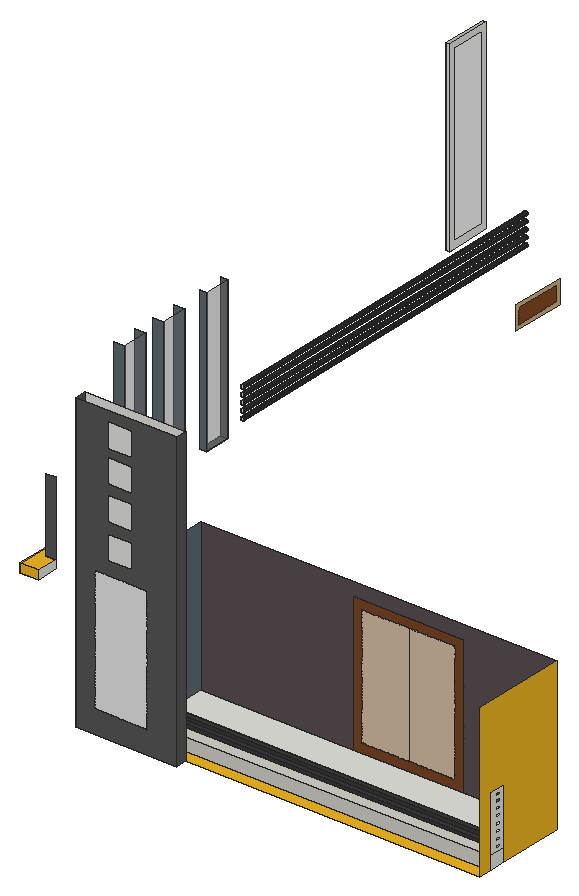
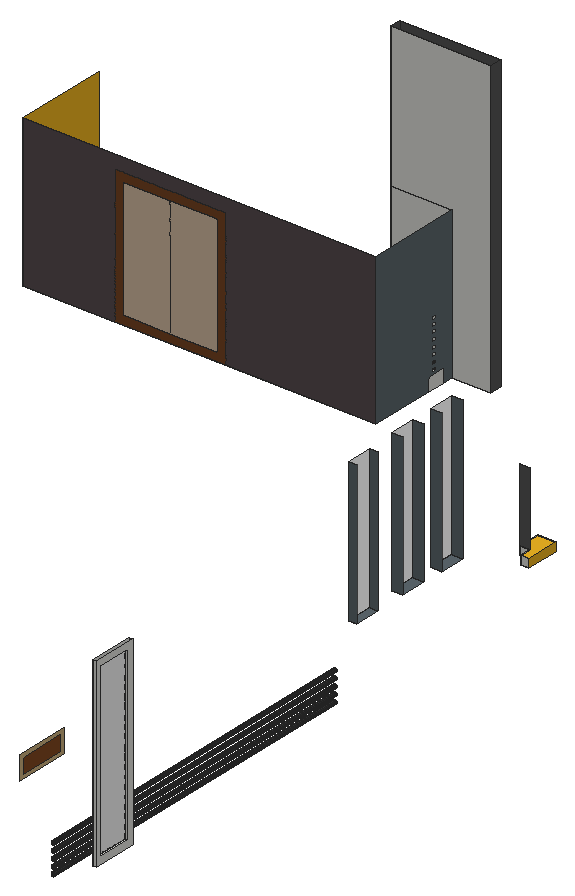
# SketchUp Ruby script. Lengths in inches.
U = 1.inch
M = Sketchup.active_model
def pt(a) = Geom::Point3d.new(a.map { |v| v * U })
def face(e, loops, mat)
  f = e.add_face(loops[0].map { |a| pt(a) })
  loops[1..].each { |l| e.add_face(l.map { |a| pt(a) }).erase! }
  f.material = f.back_material = mat if mat
  f
end
# faces: each face lists its corners as indices into pts; further lists are holes
def faces(e, pts, list, mat = nil) = list.each { |f| face(e, (f[0].is_a?(Array) ? f : [f]).map { |l| l.map { |i| pts[i] } }, mat) }
# xy, xz, yz: faces in a plane at the given z, y or x. An outline is a flat list of corners, or four numbers for a rectangle; further outlines are holes
def ring(l) = l.size == 4 ? [[l[0], l[1]], [l[2], l[1]], [l[2], l[3]], [l[0], l[3]]] : l.each_slice(2).to_a
def flat(e, list, mat, &to3) = list.each { |f| face(e, (f[0].is_a?(Array) ? f : [f]).map { |l| ring(l).map { |u, v| to3.(u, v) } }, mat) }
def xy(e, z, list, mat = nil) = flat(e, list, mat) { |x, y| [x, y, z] }
def xz(e, y, list, mat = nil) = flat(e, list, mat) { |x, z| [x, y, z] }
def yz(e, x, list, mat = nil) = flat(e, list, mat) { |y, z| [x, y, z] }
def lines(e, pts, list) = list.each { |a, b| e.add_line(pt(pts[a]), pt(pts[b])) }
# prism: a flat outline (further loops are holes) pulled along v
def prism(e, loops, v, mat = nil)
  f = face(e, loops, mat); d = Geom::Vector3d.new(v.map { |x| x * U })
  f.pushpull(f.normal.samedirection?(d) ? d.length : -d.length)
end
def box(e, o, s, mat = nil) = prism(e, [[o, [o[0] + s[0], o[1], o[2]], [o[0] + s[0], o[1] + s[1], o[2]], [o[0], o[1] + s[1], o[2]]]], [0, 0, s[2]], mat)
def at(x, y, z, deg = 0) = Geom::Transformation.translation(pt([x, y, z])) * Geom::Transformation.rotation(ORIGIN, Z_AXIS, deg.degrees)
def axes(o, x, y, z) = Geom::Transformation.new([*x, 0, *y, 0, *z, 0, *pt(o).to_a, 1])
def part(name) = M.definitions.add(name)
# library, detail: a bought-in or finely detailed component or shape, given as its bounding box
def library(name, o, s) = part(name).tap { |d| box(d.entities, o, s) }
def detail(e, o, s) = box(e.add_group.entities, o, s)
def put(e, d, t, mat = nil) = e.add_instance(d, t).tap { |i| i.material = mat if mat }
def group(e, t, mat = nil) = e.add_group.tap { |g| g.transformation = t; g.material = mat if mat }.entities
root = M.entities
M.materials.add("[0045_Goldenrod]").color = [239, 181, 35]
M.materials.add("[Asphalt New]").color = [89, 79, 82]
M.materials.add("[Color M06]").color = [86, 86, 86]
M.materials.add("[Color M07]").color = [58, 58, 58]
M.materials.add("[Formica Laminate Light]").color = [213, 189, 164]
M.materials.add("[Formica Speckled Grey]").color = [94, 105, 111]
M.materials.add("[Sketchy Siding Scale]").color = [229, 229, 229]
M.materials.add("[Sketchy Siding Scale]1").color = [244, 244, 244]
M.materials.add("[Tile Travertine 2 inch]").color = [211, 208, 201]
M.materials.add("[Translucent Glass Gray]1").color = [128, 128, 128]
M.materials["[Translucent Glass Gray]1"].alpha = 0.5
M.materials.add("[Wood Cherry Original]").color = [130, 73, 35]
M.materials.add("[Wood Floor Light]").color = [204, 176, 127]
M.materials.add("[Wood Veneer 01]1").color = [120, 70, 37]
xy(root,228.72,[[38.625,253.03,38.625,280.03,45.3125,280.03,45.3125,270.46,53.375,270.46,53.375,253.03]],"[0045_Goldenrod]")
xy(root,232.59,[[226.34,133.21,513.45,147.47],[226.34,147.47,513.45,200.74]])
xy(root,232.59,[[226.34,123.625,513.45,133.21]],"[0045_Goldenrod]")
xy(root,232.59,[[194.63,114.1875,276.16,123.625]],"[Color M06]")
xy(root,235.53,[[38.625,253.03,53.375,253.03,53.375,270.46,45.3125,270.46,45.3125,280.03,38.625,280.03]],"[0045_Goldenrod]")
xy(root,238.4,[[0,731.17,2.5625,767.73]])
xy(root,242.9,[[226.34,133.21,513.45,147.47]],"[Tile Travertine 2 inch]")
xy(root,244.23,[[0,735.45,2.5625,763.82]])
xy(root,245.27,[[226.34,139.81,513.45,143.95]])
xy(root,247.83,[[226.34,139.81,513.45,143.95]],"[Color M07]")
xy(root,250.64,[[226.34,139.81,513.45,143.95]])
xy(root,251.86,[[53.375,329.31,62.1875,350.56],[53.375,368.62,61.9375,389.87],[53.375,415.62,59.375,436.87]],"[Formica Speckled Grey]")
xy(root,253.2,[[226.34,139.81,513.45,143.95]],"[Color M07]")
xz(root,114.1875,[[[194.63,232.59,276.16,471],[209.79,250.99,251.85,351.68],[220.22,443.22,239.85,462.84],[220.22,362.15,239.85,381.78],[220.22,417.34,239.85,436.97],[220.22,390.15,239.85,409.78]]],"[Color M06]")
xz(root,114.1875,[[209.79,250.99,251.85,351.68]],"[Sketchy Siding Scale]")
xz(root,123.625,[[194.63,232.59,194.63,471,276.16,471,276.16,354.51,226.34,354.51,226.34,232.59],[226.34,232.59,276.16,354.51]])
xz(root,133.21,[[226.34,232.59,513.45,242.9]],"[Tile Travertine 2 inch]")
xz(root,139.81,[[226.34,245.27,513.45,247.83],[226.34,250.64,513.45,253.2]],"[Color M07]")
xz(root,143.95,[[226.34,245.27,513.45,247.83],[226.34,250.64,513.45,253.2]])
xz(root,147.47,[[226.34,232.59,513.45,242.9]])
xz(root,200.74,[[226.34,232.59,348.83,232.59,348.83,343.46,438.71,343.46,438.71,232.59,513.45,232.59,513.45,354.51,226.34,354.51]],"[Asphalt New]")
xz(root,200.74,[[355.93,239.69,393.77,336.36],[393.77,239.69,431.6,336.36]],"[Formica Laminate Light]")
xz(root,200.74,[[[348.83,232.59,438.71,343.46],[355.93,239.69,431.6,336.36]]],"[Wood Veneer 01]1")
xz(root,253.03,[[38.625,228.72,53.375,235.53]],"[0045_Goldenrod]")
xz(root,270.46,[[45.3125,228.72,53.375,235.53]])
xz(root,270.46,[[45.3125,235.53,53.375,295.16]],"[Color M06]")
xz(root,280.03,[[38.625,228.72,45.3125,235.53]])
xz(root,329.31,[[53.375,251.86,62.1875,367.23]],"[Formica Speckled Grey]")
xz(root,350.56,[[53.375,251.86,62.1875,367.23]],"[Formica Speckled Grey]")
xz(root,368.62,[[53.375,251.86,61.9375,367.23]],"[Formica Speckled Grey]")
xz(root,389.87,[[53.375,251.86,61.9375,367.23]],"[Formica Speckled Grey]")
xz(root,415.62,[[53.375,251.86,59.375,367.23]],"[Formica Speckled Grey]")
xz(root,436.87,[[53.375,251.86,59.375,367.23]],"[Formica Speckled Grey]")
xz(root,493.85,[[25.42,228.28,25.79,228.33,26.14,228.48,26.4375,228.71,26.66,229,26.81,229.35,26.86,229.72,26.81,230.09,26.66,230.44,26.4375,230.74,26.14,230.97,25.79,231.11,25.42,231.16,25.05,231.11,24.7,230.97,24.4,230.74,24.17,230.44,24.03,230.09,23.98,229.72,24.03,229.35,24.17,229,24.4,228.71,24.7,228.48,25.05,228.33],[25.42,233.97,25.79,234.02,26.14,234.16,26.4375,234.39,26.66,234.69,26.81,235.04,26.86,235.41,26.81,235.78,26.66,236.13,26.4375,236.43,26.14,236.65,25.79,236.8,25.42,236.85,25.05,236.8,24.7,236.65,24.4,236.43,24.17,236.13,24.03,235.78,23.98,235.41,24.03,235.04,24.17,234.69,24.4,234.39,24.7,234.16,25.05,234.02],[25.42,239.53,25.79,239.58,26.14,239.73,26.4375,239.96,26.66,240.25,26.81,240.6,26.86,240.97,26.81,241.34,26.66,241.69,26.4375,241.99,26.14,242.22,25.79,242.36,25.42,242.41,25.05,242.36,24.7,242.22,24.4,241.99,24.17,241.69,24.03,241.34,23.98,240.97,24.03,240.6,24.17,240.25,24.4,239.96,24.7,239.73,25.05,239.58],[25.42,245.53,25.79,245.58,26.14,245.73,26.4375,245.96,26.66,246.25,26.81,246.6,26.86,246.97,26.81,247.34,26.66,247.69,26.4375,247.99,26.14,248.22,25.79,248.36,25.42,248.41,25.05,248.36,24.7,248.22,24.4,247.99,24.17,247.69,24.03,247.34,23.98,246.97,24.03,246.6,24.17,246.25,24.4,245.96,24.7,245.73,25.05,245.58],[25.42,251.22,25.79,251.27,26.14,251.41,26.4375,251.64,26.66,251.94,26.81,252.29,26.86,252.66,26.81,253.03,26.66,253.38,26.4375,253.68,26.14,253.9,25.79,254.05,25.42,254.1,25.05,254.05,24.7,253.9,24.4,253.68,24.17,253.38,24.03,253.03,23.98,252.66,24.03,252.29,24.17,251.94,24.4,251.64,24.7,251.41,25.05,251.27]])
xz(root,731.17,[[0,238.4,2.5625,388.58]])
xz(root,735.45,[[0,244.23,2.5625,383.48]])
xz(root,763.82,[[0,244.23,2.5625,383.48]])
xz(root,767.73,[[0,238.4,2.5625,388.58]])
yz(root,0,[[[731.17,238.4,767.73,388.58],[735.45,244.23,763.82,383.48]]])
yz(root,2.5625,[[[731.17,238.4,767.73,388.58],[735.45,244.23,763.82,383.48]]])
yz(root,2.5625,[[735.45,244.23,763.82,383.48]],"[Sketchy Siding Scale]1")
yz(root,38.625,[[253.03,228.72,280.03,235.53]],"[0045_Goldenrod]")
yz(root,45.3125,[[270.46,228.72,280.03,235.53]])
yz(root,53.375,[[253.03,228.72,270.46,235.53]])
yz(root,59.375,[[415.62,251.86,436.87,367.23]],"[Translucent Glass Gray]1")
yz(root,61.9375,[[368.62,251.86,389.87,367.23]],"[Translucent Glass Gray]1")
yz(root,62.1875,[[329.31,251.86,350.56,367.23]],"[Translucent Glass Gray]1")
yz(root,103.59,[[675.22,245.69,712.4,257.5625]],"[Wood Cherry Original]")
yz(root,103.59,[[[671.74,242.22,715.87,261.03],[675.22,245.69,712.4,257.5625]]],"[Wood Floor Light]")
yz(root,194.63,[[114.1875,232.59,123.625,471]],"[Color M06]")
yz(root,226.34,[[133.21,232.59,147.47,242.9]])
yz(root,226.34,[[[123.625,232.59,133.21,232.59,133.21,242.9,147.47,242.9,147.47,232.59,200.74,232.59,200.74,354.51,123.625,354.51],[139.81,245.27,143.95,247.83],[139.81,250.64,143.95,253.2],[139.81,256.33,143.95,258.89],[139.81,261.64,143.95,264.2],[139.81,267.45,143.95,270.02],[139.81,273.08,143.95,275.64],[139.81,278.27,143.95,280.83],[139.81,283.14,143.95,285.7]]],"[Formica Speckled Grey]")
yz(root,276.16,[[114.1875,232.59,123.625,471]],"[Color M06]")
yz(root,513.45,[[133.21,232.59,147.47,242.9],[[133.21,242.9,147.47,288.46],[139.81,283.14,143.95,285.7],[139.81,245.27,143.95,247.83],[139.81,278.27,143.95,280.83],[139.81,250.64,143.95,253.2],[139.81,273.08,143.95,275.64],[139.81,256.33,143.95,258.89],[139.81,267.45,143.95,270.02],[139.81,261.64,143.95,264.2]],[139.81,245.27,143.95,247.83],[139.81,250.64,143.95,253.2]])
yz(root,513.45,[[123.625,232.59,123.625,354.51,200.74,354.51,200.74,232.59,147.47,232.59,147.47,288.46,133.21,288.46,133.21,232.59]],"[0045_Goldenrod]")
p = [[25.05,493.85,228.33],[24.7,493.85,228.48],[24.7,779.875,228.48],[25.05,779.875,228.33],[25.42,493.85,228.28],[25.42,779.875,228.28],
  [25.79,493.85,228.33],[25.79,779.875,228.33],[26.14,493.85,228.48],[26.14,779.875,228.48],[24.4,493.85,228.71],[24.4,779.875,228.71],
  [26.4375,493.85,228.71],[26.4375,779.875,228.71],[24.17,493.85,229],[24.17,779.875,229],[26.66,493.85,229],[26.66,779.875,229],
  [24.03,493.85,229.35],[24.03,779.875,229.35],[26.81,493.85,229.35],[26.81,779.875,229.35],[23.98,493.85,229.72],[23.98,779.875,229.72],
  [26.86,493.85,229.72],[26.86,779.875,229.72],[24.03,493.85,230.09],[24.03,779.875,230.09],[26.81,493.85,230.09],[26.81,779.875,230.09],
  [24.17,493.85,230.44],[24.17,779.875,230.44],[26.66,493.85,230.44],[26.66,779.875,230.44],[24.4,493.85,230.74],[24.4,779.875,230.74],
  [26.4375,493.85,230.74],[26.4375,779.875,230.74],[24.7,493.85,230.97],[24.7,779.875,230.97],[26.14,493.85,230.97],[26.14,779.875,230.97],
  [25.05,493.85,231.11],[25.05,779.875,231.11],[25.79,493.85,231.11],[25.79,779.875,231.11],[25.42,493.85,231.16],[25.42,779.875,231.16],
  [25.05,493.85,234.02],[24.7,493.85,234.16],[24.7,779.875,234.16],[25.05,779.875,234.02],[25.42,493.85,233.97],[25.42,779.875,233.97],
  [25.79,493.85,234.02],[25.79,779.875,234.02],[26.14,493.85,234.16],[26.14,779.875,234.16],[24.4,493.85,234.39],[24.4,779.875,234.39],
  [26.4375,493.85,234.39],[26.4375,779.875,234.39],[24.17,493.85,234.69],[24.17,779.875,234.69],[26.66,493.85,234.69],[26.66,779.875,234.69],
  [24.03,493.85,235.04],[24.03,779.875,235.04],[26.81,493.85,235.04],[26.81,779.875,235.04],[23.98,493.85,235.41],[23.98,779.875,235.41],
  [26.86,493.85,235.41],[26.86,779.875,235.41],[24.03,493.85,235.78],[24.03,779.875,235.78],[26.81,493.85,235.78],[26.81,779.875,235.78],
  [24.17,493.85,236.13],[24.17,779.875,236.13],[26.66,493.85,236.13],[26.66,779.875,236.13],[24.4,493.85,236.43],[24.4,779.875,236.43],
  [26.4375,493.85,236.43],[26.4375,779.875,236.43],[24.7,493.85,236.65],[24.7,779.875,236.65],[26.14,493.85,236.65],[26.14,779.875,236.65],
  [25.05,493.85,236.8],[25.05,779.875,236.8],[25.79,493.85,236.8],[25.79,779.875,236.8],[25.42,493.85,236.85],[25.42,779.875,236.85],
  [25.42,493.85,239.53],[25.05,493.85,239.58],[25.05,779.875,239.58],[25.42,779.875,239.53],[25.79,493.85,239.58],[25.79,779.875,239.58],
  [24.7,493.85,239.73],[24.7,779.875,239.73],[26.14,493.85,239.73],[26.14,779.875,239.73],[24.4,493.85,239.96],[24.4,779.875,239.96],
  [26.4375,493.85,239.96],[26.4375,779.875,239.96],[24.17,493.85,240.25],[24.17,779.875,240.25],[26.66,493.85,240.25],[26.66,779.875,240.25],
  [24.03,493.85,240.6],[24.03,779.875,240.6],[26.81,493.85,240.6],[26.81,779.875,240.6],[23.98,493.85,240.97],[23.98,779.875,240.97],
  [26.86,493.85,240.97],[26.86,779.875,240.97],[24.03,493.85,241.34],[24.03,779.875,241.34],[26.81,493.85,241.34],[26.81,779.875,241.34],
  [24.17,493.85,241.69],[24.17,779.875,241.69],[26.66,493.85,241.69],[26.66,779.875,241.69],[24.4,493.85,241.99],[24.4,779.875,241.99],
  [26.4375,493.85,241.99],[26.4375,779.875,241.99],[24.7,493.85,242.22],[24.7,779.875,242.22],[26.14,493.85,242.22],[26.14,779.875,242.22],
  [25.05,493.85,242.36],[25.05,779.875,242.36],[25.79,493.85,242.36],[25.79,779.875,242.36],[25.42,493.85,242.41],[25.42,779.875,242.41],
  [25.42,493.85,245.53],[25.05,493.85,245.58],[25.05,779.875,245.58],[25.42,779.875,245.53],[25.79,493.85,245.58],[25.79,779.875,245.58],
  [24.7,493.85,245.73],[24.7,779.875,245.73],[26.14,493.85,245.73],[26.14,779.875,245.73],[24.4,493.85,245.96],[24.4,779.875,245.96],
  [26.4375,493.85,245.96],[26.4375,779.875,245.96],[24.17,493.85,246.25],[24.17,779.875,246.25],[26.66,493.85,246.25],[26.66,779.875,246.25],
  [24.03,493.85,246.6],[24.03,779.875,246.6],[26.81,493.85,246.6],[26.81,779.875,246.6],[23.98,493.85,246.97],[23.98,779.875,246.97],
  [26.86,493.85,246.97],[26.86,779.875,246.97],[24.03,493.85,247.34],[24.03,779.875,247.34],[26.81,493.85,247.34],[26.81,779.875,247.34],
  [24.17,493.85,247.69],[24.17,779.875,247.69],[26.66,493.85,247.69],[26.66,779.875,247.69],[24.4,493.85,247.99],[24.4,779.875,247.99],
  [26.4375,493.85,247.99],[26.4375,779.875,247.99],[24.7,493.85,248.22],[24.7,779.875,248.22],[26.14,493.85,248.22],[26.14,779.875,248.22],
  [25.05,493.85,248.36],[25.05,779.875,248.36],[25.79,493.85,248.36],[25.79,779.875,248.36],[25.42,493.85,248.41],[25.42,779.875,248.41],
  [25.42,493.85,251.22],[25.05,493.85,251.27],[25.05,779.875,251.27],[25.42,779.875,251.22],[25.79,493.85,251.27],[25.79,779.875,251.27],
  [24.7,493.85,251.41],[24.7,779.875,251.41],[26.14,493.85,251.41],[26.14,779.875,251.41],[24.4,493.85,251.64],[24.4,779.875,251.64],
  [26.4375,493.85,251.64],[26.4375,779.875,251.64],[24.17,493.85,251.94],[24.17,779.875,251.94],[26.66,493.85,251.94],[26.66,779.875,251.94],
  [24.03,493.85,252.29],[24.03,779.875,252.29],[26.81,493.85,252.29],[26.81,779.875,252.29],[23.98,493.85,252.66],[23.98,779.875,252.66],
  [26.86,493.85,252.66],[26.86,779.875,252.66],[24.03,493.85,253.03],[24.03,779.875,253.03],[26.81,493.85,253.03],[26.81,779.875,253.03],
  [24.17,493.85,253.38],[24.17,779.875,253.38],[26.66,493.85,253.38],[26.66,779.875,253.38],[24.4,493.85,253.68],[24.4,779.875,253.68],
  [26.4375,493.85,253.68],[26.4375,779.875,253.68],[24.7,493.85,253.9],[24.7,779.875,253.9],[26.14,493.85,253.9],[26.14,779.875,253.9],
  [25.05,493.85,254.05],[25.05,779.875,254.05],[25.79,493.85,254.05],[25.79,779.875,254.05],[25.42,493.85,254.1],[25.42,779.875,254.1]]
faces(root,p,[[0,1,2,3],[4,0,3,5],[6,4,5,7],[8,6,7,9],[1,10,11,2],[12,8,9,13],[10,14,15,11],[16,12,13,17],
  [14,18,19,15],[20,16,17,21],[18,22,23,19],[24,20,21,25],[22,26,27,23],[28,24,25,29],[26,30,31,27],[32,28,29,33],
  [30,34,35,31],[36,32,33,37],[34,38,39,35],[40,36,37,41],[38,42,43,39],[44,40,41,45],[42,46,47,43],[46,44,45,47],
  [48,49,50,51],[52,48,51,53],[54,52,53,55],[56,54,55,57],[49,58,59,50],[60,56,57,61],[58,62,63,59],[64,60,61,65],
  [62,66,67,63],[68,64,65,69],[66,70,71,67],[72,68,69,73],[70,74,75,71],[76,72,73,77],[74,78,79,75],[80,76,77,81],
  [78,82,83,79],[84,80,81,85],[82,86,87,83],[88,84,85,89],[86,90,91,87],[92,88,89,93],[90,94,95,91],[94,92,93,95],
  [96,97,98,99],[100,96,99,101],[97,102,103,98],[104,100,101,105],[102,106,107,103],[108,104,105,109],[106,110,111,107],[112,108,109,113],
  [110,114,115,111],[116,112,113,117],[114,118,119,115],[120,116,117,121],[118,122,123,119],[124,120,121,125],[122,126,127,123],[128,124,125,129],
  [126,130,131,127],[132,128,129,133],[130,134,135,131],[136,132,133,137],[134,138,139,135],[140,136,137,141],[138,142,143,139],[142,140,141,143],
  [144,145,146,147],[148,144,147,149],[145,150,151,146],[152,148,149,153],[150,154,155,151],[156,152,153,157],[154,158,159,155],[160,156,157,161],
  [158,162,163,159],[164,160,161,165],[162,166,167,163],[168,164,165,169],[166,170,171,167],[172,168,169,173],[170,174,175,171],[176,172,173,177],
  [174,178,179,175],[180,176,177,181],[178,182,183,179],[184,180,181,185],[182,186,187,183],[188,184,185,189],[186,190,191,187],[190,188,189,191],
  [192,193,194,195],[196,192,195,197],[193,198,199,194],[200,196,197,201],[198,202,203,199],[204,200,201,205],[202,206,207,203],[208,204,205,209],
  [206,210,211,207],[212,208,209,213],[210,214,215,211],[216,212,213,217],[214,218,219,215],[220,216,217,221],[218,222,223,219],[224,220,221,225],
  [222,226,227,223],[228,224,225,229],[226,230,231,227],[232,228,229,233],[230,234,235,231],[236,232,233,237],[234,238,239,235],[238,236,237,239]],"[Color M07]")
